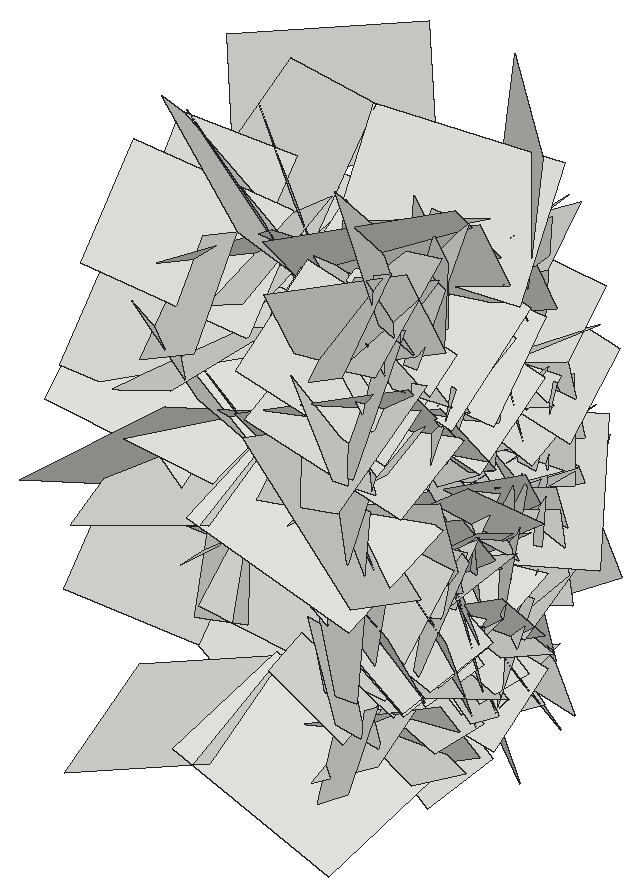
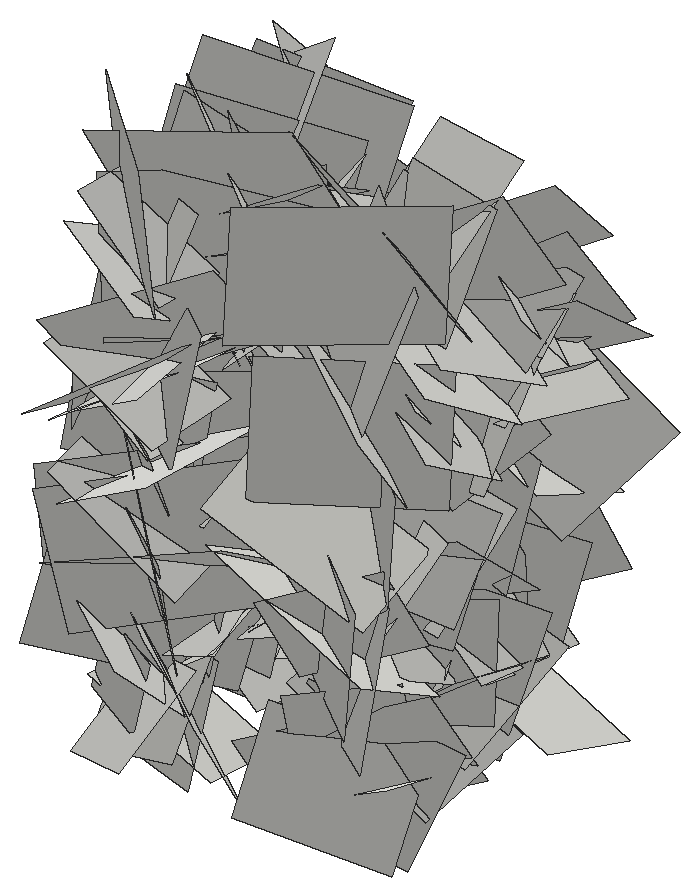
# SketchUp Ruby script. Lengths in inches.
U = 1.inch
M = Sketchup.active_model
def pt(a) = Geom::Point3d.new(a.map { |v| v * U })
def face(e, loops, mat)
  f = e.add_face(loops[0].map { |a| pt(a) })
  loops[1..].each { |l| e.add_face(l.map { |a| pt(a) }).erase! }
  f.material = f.back_material = mat if mat
  f
end
# faces: each face lists its corners as indices into pts; further lists are holes
def faces(e, pts, list, mat = nil) = list.each { |f| face(e, (f[0].is_a?(Array) ? f : [f]).map { |l| l.map { |i| pts[i] } }, mat) }
# xy, xz, yz: faces in a plane at the given z, y or x. An outline is a flat list of corners, or four numbers for a rectangle; further outlines are holes
def ring(l) = l.size == 4 ? [[l[0], l[1]], [l[2], l[1]], [l[2], l[3]], [l[0], l[3]]] : l.each_slice(2).to_a
def flat(e, list, mat, &to3) = list.each { |f| face(e, (f[0].is_a?(Array) ? f : [f]).map { |l| ring(l).map { |u, v| to3.(u, v) } }, mat) }
def xy(e, z, list, mat = nil) = flat(e, list, mat) { |x, y| [x, y, z] }
def xz(e, y, list, mat = nil) = flat(e, list, mat) { |x, z| [x, y, z] }
def yz(e, x, list, mat = nil) = flat(e, list, mat) { |y, z| [x, y, z] }
def lines(e, pts, list) = list.each { |a, b| e.add_line(pt(pts[a]), pt(pts[b])) }
# prism: a flat outline (further loops are holes) pulled along v
def prism(e, loops, v, mat = nil)
  f = face(e, loops, mat); d = Geom::Vector3d.new(v.map { |x| x * U })
  f.pushpull(f.normal.samedirection?(d) ? d.length : -d.length)
end
def box(e, o, s, mat = nil) = prism(e, [[o, [o[0] + s[0], o[1], o[2]], [o[0] + s[0], o[1] + s[1], o[2]], [o[0], o[1] + s[1], o[2]]]], [0, 0, s[2]], mat)
def at(x, y, z, deg = 0) = Geom::Transformation.translation(pt([x, y, z])) * Geom::Transformation.rotation(ORIGIN, Z_AXIS, deg.degrees)
def axes(o, x, y, z) = Geom::Transformation.new([*x, 0, *y, 0, *z, 0, *pt(o).to_a, 1])
def part(name) = M.definitions.add(name)
# library, detail: a bought-in or finely detailed component or shape, given as its bounding box
def library(name, o, s) = part(name).tap { |d| box(d.entities, o, s) }
def detail(e, o, s) = box(e.add_group.entities, o, s)
def put(e, d, t, mat = nil) = e.add_instance(d, t).tap { |i| i.material = mat if mat }
def group(e, t, mat = nil) = e.add_group.tap { |g| g.transformation = t; g.material = mat if mat }.entities
root = M.entities
c1 = part("Component\#6")
p = [[0.01,0,0],[0,3.24,4.54],[4.32,3.24,4.54],[4.33,0,0]]
faces(c1.entities,p,[[0,1,2,3]])
put(root,c1,axes([14.53,167.01,8.33],[0.18631,0.3359,0.73427],[0.04897,0.74605,-0.35235],[0.8545,-0.11599,-0.1399]))
put(root,c1,axes([14.53,166.18,19.56],[-0.12535,0.0531,1.28965],[-0.2192,1.27754,-0.07157],[1.35051,0.21229,0.10808]))
put(root,c1,axes([14.53,168.14,0.12],[-0.06773,-0.63363,0.78179],[0.11595,0.77435,0.63654],[1.06038,-0.12515,-0.01967]))
put(root,c1,axes([14.53,169.19,10.7],[-0.0913,0.46499,-1.24639],[-0.29576,-1.22753,-0.43867],[1.37875,-0.23253,-0.17663]))
put(root,c1,axes([18.5,165.96,10.85],[0.09912,0.20412,-0.70693],[0.02587,-0.71308,-0.20267],[-0.77953,0.00229,-0.09661]))
put(root,c1,axes([18.5,161.25,17.66],[0.25985,0.898,-0.37026],[0.14737,-0.41038,-0.90325],[-1.01902,0.16964,-0.22504]))
put(root,c1,axes([18.5,162.79,15.86],[0.07285,0.46729,0.4905],[-0.02436,0.49435,-0.46773],[-0.71769,0.03066,0.06566]))
put(root,c1,axes([14.53,167.22,15.375],[-0.0235,-0.92066,-0.53568],[-0.01768,-0.53543,0.92093],[1.12894,-0.02755,0.00327]))
put(root,c1,axes([14.53,167.28,17.92],[-0.19972,-0.96368,-0.57877],[0.14667,-0.60226,0.95775],[1.18251,-0.08806,-0.21655]))
put(root,c1,axes([14.53,157.18,19.73],[-0.07599,0.81527,0.8297],[-0.084,0.82592,-0.8184],[1.23014,0.10676,-0.00463]))
put(root,c1,axes([14.53,167.18,1.59],[-0.07507,-1.0991,0.32301],[-0.05871,0.32653,1.09895],[1.2129,-0.05222,0.07319]))
put(root,c1,axes([14.53,168.87,14.79],[0.03205,0.06087,-1.12787],[-0.16204,-1.11767,-0.06442],[1.18627,-0.15431,0.02167]))
put(root,c1,axes([14.53,166.01,11.8],[0.21466,0.53877,-0.68228],[-0.03009,-0.69607,-0.55809],[0.92102,-0.14831,0.14079]))
put(root,c1,axes([14.53,163.57,3.71],[0.11292,-0.2033,0.99476],[-0.09749,0.99417,0.21302],[1.07181,0.11185,-0.08542]))
put(root,c1,axes([14.53,159.91,9.22],[-0.2022,-1.20502,0.50539],[-0.1049,0.52261,1.20871],[1.38114,-0.13672,0.1658]))
put(root,c1,axes([14.53,162.44,14.8125],[-0.22172,-1.13603,-0.19278],[0.19013,-0.22565,1.13507],[1.20652,-0.17321,-0.21429]))
put(root,c1,axes([14.53,160.62,5.12],[0.08568,1.04485,0.18773],[-0.09569,0.19436,-1.04286],[1.1212,-0.06325,-0.10335]))
put(root,c1,axes([18.5,162.91,7.6875],[0.03517,0.6334,0.29771],[0.1292,0.28826,-0.62688],[-0.73053,0.08147,-0.09654]))
put(root,c1,axes([14.53,163.93,5.47],[0.11462,-1.01834,-0.26907],[-0.10191,-0.2789,1.0169],[1.11183,0.07941,0.12095]))
put(root,c1,axes([14.53,156.14,6.5],[0.17845,0.35117,0.84391],[0.01887,0.85668,-0.36003],[0.96872,-0.08137,-0.14844]))
put(root,c1,axes([18.5,170.02,6.34],[0.13634,-0.30577,-0.6303],[0.02329,-0.63876,0.31436],[-0.74222,-0.07621,-0.10592]))
put(root,c1,axes([14.53,160.14,4.78],[0.03826,-0.47304,0.81506],[0.18962,0.80427,0.45886],[0.98077,-0.13704,-0.12051]))
put(root,c1,axes([14.53,166.625,12.7],[0.17127,1.04033,-0.10676],[-0.13463,-0.08771,-1.04688],[1.10034,-0.17266,-0.11147]))
put(root,c1,axes([14.53,168.99,0.33],[0.20008,-0.71049,0.66963],[-0.07161,0.67089,0.73087],[1.03242,0.18422,-0.07908]))
put(root,c1,axes([14.53,164.18,5.53],[0.00871,-1.21515,-0.1589],[-0.11926,-0.15898,1.20995],[1.29354,-0.00648,0.11262]))
put(root,c1,axes([18.5,159.77,13.93],[0.14822,0.47929,0.38572],[-0.01533,0.39801,-0.48932],[-0.65196,0.0996,0.0992]))
put(root,c1,axes([14.53,165.6875,8.33],[0.14254,-0.77018,0.64298],[0.05856,0.65343,0.77114],[1.06187,0.06735,-0.12884]))
put(root,c1,axes([14.53,164.53,2.65],[0.11418,0.95876,0.15487],[0.16789,0.13639,-0.95453],[1.01568,-0.13033,0.14037]))
put(root,c1,axes([14.53,170.79,17.67],[0.07972,-0.69903,-0.88266],[-0.01234,-0.88506,0.69994],[1.19343,0.03754,0.0662]))
put(root,c1,axes([14.53,165.97,13.03],[0.11695,-0.23373,1.15092],[-0.10796,1.14973,0.24325],[1.24018,0.12213,-0.08736]))
put(root,c1,axes([18.5,164.09,3.1],[0.16189,-0.51758,0.36968],[0.06161,0.38995,0.52196],[-0.67139,-0.08902,0.13704]))
put(root,c1,axes([14.53,155.93,16.01],[0.06166,0.77521,1.08886],[-0.24821,1.07895,-0.75564],[1.39492,0.15772,-0.18259]))
put(root,c1,axes([14.53,163.21,2.24],[-0.08398,-0.53221,1.10764],[0.11648,1.10243,0.53756],[1.29738,-0.13342,0.02343]))
put(root,c1,axes([14.53,161.02,12.77],[0.04866,0.36936,-1.04237],[0.12613,-1.03886,-0.36288],[1.16543,0.09701,0.0828]))
put(root,c1,axes([14.53,162.03,18.62],[0.15865,-0.78055,-0.79386],[-0.03617,-0.80384,0.78393],[1.17956,0.08034,0.13081]))
put(root,c1,axes([14.53,161.03,16.77],[-0.02327,0.73455,-0.90907],[0.17416,-0.89826,-0.72978],[1.22657,0.14148,0.08637]))
put(root,c1,axes([14.53,163.86,1.73],[0.03729,0.66749,1.03354],[-0.00972,1.03407,-0.66752],[1.30413,-0.01138,-0.03452]))
put(root,c1,axes([14.53,162.85,15.75],[0.04254,-1.00522,0.67204],[0.02385,0.67292,1.00519],[1.28151,0.02084,-0.04102]))
put(root,c1,axes([14.53,163.36,23.49],[0.04873,0.57368,-1.00395],[0.12423,-1.00188,-0.56714],[1.21936,0.07915,0.09791]))
put(root,c1,axes([14.53,159.69,18.96],[0.02704,0.74145,1.09535],[-0.09362,1.09406,-0.73853],[1.39894,0.05888,-0.07059]))
put(root,c1,axes([14.53,166.4,18.65],[-0.092,-1.19571,-0.63762],[0.0325,-0.6405,1.19693],[1.43603,-0.06211,-0.06794]))
put(root,c1,axes([14.53,155.03,14.95],[-0.10989,1.07322,0.82249],[0.07177,0.82799,-1.07186],[1.43147,0.04087,0.11688]))
put(root,c1,axes([14.53,159.14,18.38],[0.07521,0.79304,-0.86536],[0.12573,-0.86735,-0.78513],[1.23784,0.03991,0.13233]))
put(root,c1,axes([14.53,168.375,23.9],[-0.0952,-0.72561,-1.04974],[0.29336,-1.03837,0.69407],[1.32049,0.17837,-0.22987]))
put(root,c1,axes([14.53,157.93,15.34],[0.27083,1.19165,0.15594],[-0.0802,0.17506,-1.21378],[1.27139,-0.2428,-0.10978]))
put(root,c1,axes([14.53,162.31,11.53],[0.17206,0.75955,-0.87532],[0.12131,-0.89005,-0.75111],[1.22246,-0.01858,0.19774]))
put(root,c1,axes([14.53,165.1,2.71],[-0.06092,-1.21711,0.58199],[0.18306,0.57109,1.21136],[1.41828,-0.12599,-0.13136]))
put(root,c1,axes([14.53,170.58,10.37],[0.24309,-1.14649,0.14454],[0.04952,0.15643,1.16674],[1.2239,0.22139,-0.07591]))
put(root,c1,axes([14.53,161.07,7.88],[0.0926,0.91308,0.78861],[0.24837,0.76278,-0.90913],[1.25453,-0.21841,0.12178]))
put(root,c1,axes([14.53,171.01,11.29],[0.23144,-0.15428,-1.27652],[-0.01824,-1.29503,0.15357],[1.36284,0.00887,0.21884]))
put(root,c1,axes([14.53,167.61,21.95],[0.32344,0.31012,-1.26322],[-0.1451,-1.28265,-0.34796],[1.37111,-0.2089,0.26116]))
put(root,c1,axes([14.53,161.91,24.73],[0.20116,0.87735,-0.9177],[0.06395,-0.93308,-0.87958],[1.34427,-0.0869,0.17917]))
put(root,c1,axes([14.53,161.24,11.55],[0.08722,-1.18104,-0.51149],[0.30261,-0.48302,1.16122],[1.33028,0.18731,-0.23062]))
put(root,c1,axes([14.53,160.65,1.35],[0.1594,-1.22011,-0.46707],[0.28659,-0.43091,1.2127],[1.35486,0.2347,-0.20157]))
put(root,c1,axes([14.53,170.67,8.29],[0.13658,-1.14766,-0.62909],[0.33753,-0.58565,1.13362],[1.34561,0.26339,-0.2205]))
put(root,c1,axes([14.53,161.87,9.58],[0.35888,-0.49511,-1.17449],[0.11741,-1.19919,0.53746],[1.34594,0.23663,0.26628]))
put(root,c1,axes([28.31,161.87,9.58],[-0.35888,-0.49511,-1.17449],[-0.11741,-1.19919,0.53746],[-1.34594,0.23663,0.26628]))
put(root,c1,axes([28.31,170.67,8.29],[-0.13658,-1.14766,-0.62909],[-0.33753,-0.58565,1.13362],[-1.34561,0.26339,-0.2205]))
put(root,c1,axes([28.31,160.65,1.35],[-0.1594,-1.22011,-0.46707],[-0.28659,-0.43091,1.2127],[-1.35486,0.2347,-0.20157]))
put(root,c1,axes([28.31,161.24,11.55],[-0.08722,-1.18104,-0.51149],[-0.30261,-0.48302,1.16122],[-1.33028,0.18731,-0.23062]))
put(root,c1,axes([28.31,161.91,24.73],[-0.20116,0.87735,-0.9177],[-0.06395,-0.93308,-0.87958],[-1.34427,-0.0869,0.17917]))
put(root,c1,axes([28.31,167.61,21.95],[-0.32344,0.31012,-1.26322],[0.1451,-1.28265,-0.34796],[-1.37111,-0.2089,0.26116]))
put(root,c1,axes([28.31,171.01,11.29],[-0.23144,-0.15428,-1.27652],[0.01824,-1.29503,0.15357],[-1.36284,0.00887,0.21884]))
put(root,c1,axes([28.31,161.07,7.88],[-0.0926,0.91308,0.78861],[-0.24837,0.76278,-0.90913],[-1.25453,-0.21841,0.12178]))
put(root,c1,axes([28.31,170.58,10.37],[-0.24309,-1.14649,0.14454],[-0.04952,0.15643,1.16674],[-1.2239,0.22139,-0.07591]))
put(root,c1,axes([28.31,165.1,2.71],[0.06092,-1.21711,0.58199],[-0.18306,0.57109,1.21136],[-1.41828,-0.12599,-0.13136]))
put(root,c1,axes([28.31,162.31,11.53],[-0.17206,0.75955,-0.87532],[-0.12131,-0.89005,-0.75111],[-1.22246,-0.01858,0.19774]))
put(root,c1,axes([28.31,157.93,15.34],[-0.27083,1.19165,0.15594],[0.0802,0.17506,-1.21378],[-1.27139,-0.2428,-0.10978]))
put(root,c1,axes([28.31,168.375,23.9],[0.0952,-0.72561,-1.04974],[-0.29336,-1.03837,0.69407],[-1.32049,0.17837,-0.22987]))
put(root,c1,axes([28.31,159.14,18.38],[-0.07521,0.79304,-0.86536],[-0.12573,-0.86735,-0.78513],[-1.23784,0.03991,0.13233]))
put(root,c1,axes([28.31,155.03,14.95],[0.10989,1.07322,0.82249],[-0.07177,0.82799,-1.07186],[-1.43147,0.04087,0.11688]))
put(root,c1,axes([28.31,166.4,18.65],[0.092,-1.19571,-0.63762],[-0.0325,-0.6405,1.19693],[-1.43603,-0.06211,-0.06794]))
put(root,c1,axes([28.31,159.69,18.96],[-0.02704,0.74145,1.09535],[0.09362,1.09406,-0.73853],[-1.39894,0.05888,-0.07059]))
put(root,c1,axes([28.31,163.36,23.49],[-0.04873,0.57368,-1.00395],[-0.12423,-1.00188,-0.56714],[-1.21936,0.07915,0.09791]))
put(root,c1,axes([28.31,162.85,15.75],[-0.04254,-1.00522,0.67204],[-0.02385,0.67292,1.00519],[-1.28151,0.02084,-0.04102]))
put(root,c1,axes([28.31,163.86,1.73],[-0.03729,0.66749,1.03354],[0.00972,1.03407,-0.66752],[-1.30413,-0.01138,-0.03452]))
put(root,c1,axes([28.31,161.03,16.77],[0.02327,0.73455,-0.90907],[-0.17416,-0.89826,-0.72978],[-1.22657,0.14148,0.08637]))
put(root,c1,axes([28.31,162.03,18.62],[-0.15865,-0.78055,-0.79386],[0.03617,-0.80384,0.78393],[-1.17956,0.08034,0.13081]))
put(root,c1,axes([28.31,161.02,12.77],[-0.04866,0.36936,-1.04237],[-0.12613,-1.03886,-0.36288],[-1.16543,0.09701,0.0828]))
put(root,c1,axes([28.31,163.21,2.24],[0.08398,-0.53221,1.10764],[-0.11648,1.10243,0.53756],[-1.29738,-0.13342,0.02343]))
put(root,c1,axes([28.31,155.93,16.01],[-0.06166,0.77521,1.08886],[0.24821,1.07895,-0.75564],[-1.39492,0.15772,-0.18259]))
put(root,c1,axes([24.34,164.09,3.1],[-0.16189,-0.51758,0.36968],[-0.06161,0.38995,0.52196],[0.67139,-0.08902,0.13704]))
put(root,c1,axes([28.31,165.97,13.03],[-0.11695,-0.23373,1.15092],[0.10796,1.14973,0.24325],[-1.24018,0.12213,-0.08736]))
put(root,c1,axes([28.31,170.79,17.67],[-0.07972,-0.69903,-0.88266],[0.01234,-0.88506,0.69994],[-1.19343,0.03754,0.0662]))
put(root,c1,axes([24.34,155.94,6.59],[-0.14653,0.65267,0.04592],[-0.0729,0.03218,-0.6644],[0.6897,0.14207,-0.06047]))
put(root,c1,axes([28.31,164.53,2.65],[-0.11418,0.95876,0.15487],[-0.16789,0.13639,-0.95453],[-1.01568,-0.13033,0.14037]))
put(root,c1,axes([28.31,165.6875,8.33],[-0.14254,-0.77018,0.64298],[-0.05856,0.65343,0.77114],[-1.06187,0.06735,-0.12884]))
put(root,c1,axes([24.34,159.77,13.93],[-0.14822,0.47929,0.38572],[0.01533,0.39801,-0.48932],[0.65196,0.0996,0.0992]))
put(root,c1,axes([28.31,164.18,5.53],[-0.00871,-1.21515,-0.1589],[0.11926,-0.15898,1.20995],[-1.29354,-0.00648,0.11262]))
put(root,c1,axes([28.31,168.99,0.33],[-0.20008,-0.71049,0.66963],[0.07161,0.67089,0.73087],[-1.03242,0.18422,-0.07908]))
put(root,c1,axes([28.31,166.625,12.7],[-0.17127,1.04033,-0.10676],[0.13463,-0.08771,-1.04688],[-1.10034,-0.17266,-0.11147]))
put(root,c1,axes([28.31,160.14,4.78],[-0.03826,-0.47304,0.81506],[-0.18962,0.80427,0.45886],[-0.98077,-0.13704,-0.12051]))
put(root,c1,axes([24.34,170.02,6.34],[-0.13634,-0.30577,-0.6303],[-0.02329,-0.63876,0.31436],[0.74222,-0.07621,-0.10592]))
put(root,c1,axes([28.31,156.14,6.5],[-0.17845,0.35117,0.84391],[-0.01887,0.85668,-0.36003],[-0.96872,-0.08137,-0.14844]))
put(root,c1,axes([28.31,163.93,5.47],[-0.11462,-1.01834,-0.26907],[0.10191,-0.2789,1.0169],[-1.11183,0.07941,0.12095]))
put(root,c1,axes([24.34,162.91,7.6875],[-0.03517,0.6334,0.29771],[-0.1292,0.28826,-0.62688],[0.73053,0.08147,-0.09654]))
put(root,c1,axes([28.31,160.62,5.12],[-0.08568,1.04485,0.18773],[0.09569,0.19436,-1.04286],[-1.1212,-0.06325,-0.10335]))
put(root,c1,axes([28.31,162.44,14.8125],[0.22172,-1.13603,-0.19278],[-0.19013,-0.22565,1.13507],[-1.20652,-0.17321,-0.21429]))
put(root,c1,axes([28.31,159.91,9.22],[0.2022,-1.20502,0.50539],[0.1049,0.52261,1.20871],[-1.38114,-0.13672,0.1658]))
put(root,c1,axes([28.31,163.57,3.71],[-0.11292,-0.2033,0.99476],[0.09749,0.99417,0.21302],[-1.07181,0.11185,-0.08542]))
put(root,c1,axes([28.31,166.01,11.8],[-0.21466,0.53877,-0.68228],[0.03009,-0.69607,-0.55809],[-0.92102,-0.14831,0.14079]))
put(root,c1,axes([28.31,168.87,14.79],[-0.03205,0.06087,-1.12787],[0.16204,-1.11767,-0.06442],[-1.18627,-0.15431,0.02167]))
put(root,c1,axes([28.31,167.18,1.59],[0.07507,-1.0991,0.32301],[0.05871,0.32653,1.09895],[-1.2129,-0.05222,0.07319]))
put(root,c1,axes([28.31,157.18,19.73],[0.07599,0.81527,0.8297],[0.084,0.82592,-0.8184],[-1.23014,0.10676,-0.00463]))
put(root,c1,axes([28.31,167.28,17.92],[0.19972,-0.96368,-0.57877],[-0.14667,-0.60226,0.95775],[-1.18251,-0.08806,-0.21655]))
put(root,c1,axes([28.31,167.22,15.375],[0.0235,-0.92066,-0.53568],[0.01768,-0.53543,0.92093],[-1.12894,-0.02755,0.00327]))
put(root,c1,axes([24.34,162.79,15.86],[-0.07285,0.46729,0.4905],[0.02436,0.49435,-0.46773],[0.71769,0.03066,0.06566]))
put(root,c1,axes([24.34,161.25,17.66],[-0.25985,0.898,-0.37026],[-0.14737,-0.41038,-0.90325],[1.01902,0.16964,-0.22504]))
put(root,c1,axes([24.34,165.96,10.85],[-0.09912,0.20412,-0.70693],[-0.02587,-0.71308,-0.20267],[0.77953,0.00229,-0.09661]))
put(root,c1,axes([28.31,169.19,10.7],[0.0913,0.46499,-1.24639],[0.29576,-1.22753,-0.43867],[-1.37875,-0.23253,-0.17663]))
put(root,c1,axes([28.31,168.14,0.12],[0.06773,-0.63363,0.78179],[-0.11595,0.77435,0.63654],[-1.06038,-0.12515,-0.01967]))
put(root,c1,axes([28.31,166.18,19.56],[0.12535,0.0531,1.28965],[0.2192,1.27754,-0.07157],[-1.35051,0.21229,0.10808]))
put(root,c1,axes([28.31,167.01,8.33],[-0.18631,0.3359,0.73427],[-0.04897,0.74605,-0.35235],[-0.8545,-0.11599,-0.1399]))
put(root,c1,axes([24.34,159.82,10.86],[-0.164,0.05549,-0.7166],[0.119,-0.72215,-0.08015],[0.75252,0.12629,-0.14349]))
put(root,c1,axes([28.31,164.72,6.23],[0.02586,0.29335,1.1723],[0.23754,1.1511,-0.29271],[-1.25874,0.22326,-0.03115]))
put(root,c1,axes([24.34,164.71,11.17],[-0.09162,-0.23701,0.75882],[-0.09076,0.76162,0.22813],[0.83777,0.05659,0.1077]))
put(root,c1,axes([24.34,167.39,12.19],[-0.06725,0.11282,-0.6237],[0.12717,-0.61335,-0.12315],[0.65971,0.12973,-0.03984]))
put(root,c1,axes([24.34,158.25,7.85],[0.01053,0.60228,-0.51533],[-0.19634,-0.49934,-0.58716],[0.81696,-0.12777,-0.13447]))
put(root,c1,axes([28.31,165.51,17.74],[-0.00528,-0.97827,-0.44464],[0.11526,-0.44282,0.97306],[-1.13321,-0.04048,0.10104]))
put(root,c1,axes([28.31,165.75,-1.09],[0.03685,-0.4153,0.96157],[0.02645,0.96216,0.41465],[-1.10996,0.00914,0.04181]))
put(root,c1,axes([28.31,167.74,3.51],[0.11337,-0.86322,0.3774],[-0.28126,0.33685,0.84566],[-0.95821,-0.201,-0.20357]))
put(root,c1,axes([28.31,161.03,4.22],[-0.00206,0.54706,-0.73945],[-0.10036,-0.73565,-0.544],[-0.96983,0.07497,0.05787]))
put(root,c1,axes([28.31,158.84,13.7],[-0.15038,-0.75335,0.50607],[0.08727,0.49942,0.76653],[-0.95804,0.16374,-0.00961]))
put(root,c1,axes([28.31,166.72,20.27],[-0.14718,0.45385,-0.66356],[-0.05291,-0.67695,-0.45256],[-0.85051,-0.03642,0.14299]))
put(root,c1,axes([24.34,158.82,19.64],[0.09205,0.73549,-0.019],[-0.17536,0.00088,-0.72213],[0.75991,-0.08889,-0.16434]))
put(root,c1,axes([28.31,169.09,13.37],[-0.12805,-0.81492,0.2825],[0.01832,0.28292,0.8235],[-0.91406,0.11983,-0.02307]))
put(root,c1,axes([24.34,159.61,12.59],[0.0897,0.16152,-0.57424],[0.01993,-0.58042,-0.16049],[0.632,-0.00462,0.08656]))
put(root,c1,axes([24.34,160.65,18.69],[0.1336,-0.1743,0.59472],[-0.06624,0.60023,0.18916],[0.65357,0.09646,-0.1024]))
put(root,c1,axes([24.34,160.54,14.42],[-0.065,-0.29459,-0.75204],[-0.0763,-0.74921,0.29935],[0.85274,-0.0895,-0.03054]))
put(root,c1,axes([24.34,161.26,10.83],[-0.08958,0.45503,-0.59155],[0.06652,-0.58889,-0.46195],[0.78829,0.10141,-0.02824]))
put(root,c1,axes([28.31,170.16,13.55],[0.14984,-1.04824,-0.22204],[-0.00627,-0.22472,1.05715],[-1.13577,-0.13705,-0.03513]))
put(root,c1,axes([24.34,160.97,6.7],[0.04912,0.73058,0.10133],[-0.09877,0.10652,-0.72536],[0.77557,-0.03271,-0.0988]))
put(root,c1,axes([28.31,163.26,10.51],[-0.09772,0.8385,-0.3881],[0.10419,-0.37892,-0.842],[-0.97385,-0.12468,-0.05114]))
put(root,c1,axes([24.34,159.79,25.07],[-0.1328,0.69586,-0.68383],[-0.18687,-0.69425,-0.67416],[1.01714,-0.03669,-0.21313]))
put(root,c1,axes([28.31,167.39,3.05],[0.22625,-1.02118,-0.283],[-0.12014,-0.30902,1.02962],[-1.11681,-0.17363,-0.16809]))
put(root,c1,axes([24.34,159.32,12.84],[0.06752,-0.16321,-0.59207],[0.0871,-0.58763,0.17083],[0.64514,0.09641,0.0389]))
put(root,c1,axes([24.34,169.73,5.36],[0.07377,0.11031,-0.61615],[0.06228,-0.61836,-0.10407],[0.66058,0.04598,0.07863]))
put(root,c1,axes([28.31,166.22,16.78],[0.0558,0.90138,-0.08554],[-0.09664,-0.07998,-0.89882],[-0.95488,0.06076,0.08597]))
put(root,c1,axes([24.34,166.8,6.58],[-0.19077,-0.84984,-0.315],[0.00737,-0.32244,0.86593],[0.9607,-0.16629,-0.0692]))
put(root,c1,axes([28.31,159.03,23.29],[0.13252,0.38295,-0.87838],[-0.10893,-0.87536,-0.39626],[-1.00987,0.14467,-0.07253]))
put(root,c1,axes([24.34,160.57,3.12],[0.03509,0.82869,0.13415],[-0.15764,0.13792,-0.81528],[0.87577,-0.00838,-0.15213]))
put(root,c1,axes([24.34,164.04,15.7],[0.03624,-0.6234,-0.24842],[0.08,-0.24359,0.62167],[0.70683,0.05954,-0.05762]))
put(root,c1,axes([28.31,170.98,12.21],[0.31631,-0.51758,-1.19288],[0.16648,-1.20059,0.56021],[-1.36826,-0.26573,-0.20761]))
put(root,c1,axes([24.34,169.83,13.22],[0.13817,-0.64015,-0.16037],[-0.03989,-0.17041,0.64965],[0.69839,0.11692,0.06883]))
put(root,c1,axes([24.34,161.46,7.67],[0.11157,-0.00104,0.59962],[0.09459,0.60203,-0.01462],[0.62852,-0.09042,-0.10424]))
put(root,c1,axes([28.31,168.08,9.41],[0.11593,0.02752,-0.90523],[-0.14705,-0.90054,-0.04413],[-0.94866,0.14295,-0.10378]))
put(root,c1,axes([24.34,169.26,18.83],[0.02849,-0.83115,-0.05333],[-0.13283,-0.05679,0.82186],[0.87278,0.01849,0.12683]))
put(root,c1,axes([24.34,165.55,15.88],[-0.02597,-0.35934,-0.67832],[0.02345,-0.67872,0.35875],[0.81334,0.00809,-0.032]))
put(root,c1,axes([24.34,167.12,21.5],[0.0656,0.35319,-0.61189],[0.00255,-0.61434,-0.35436],[0.7489,-0.02885,0.0548]))
put(root,c1,axes([28.31,164.04,2.37],[0.08884,-0.86849,0.07962],[-0.14736,0.06566,0.86256],[-0.91264,-0.09515,-0.13152]))
put(root,c1,axes([28.31,162.54,0.74],[0.05881,-0.79857,0.25436],[-0.14334,0.24305,0.79255],[-0.87675,-0.0933,-0.11251]))
put(root,c1,axes([28.31,157.37,3.29],[-0.12325,0.67494,0.21472],[-0.06797,0.20667,-0.68436],[-0.74769,-0.13004,0.02682]))
put(root,c1,axes([28.31,166.02,4.84],[0.16866,0.71959,0.68076],[-0.0323,0.69272,-0.72511],[-1.04952,0.09433,0.13172]))
put(root,c1,axes([24.34,162.4,12.14],[0.15913,-0.1111,0.71617],[-0.10617,0.72117,0.13287],[0.76084,0.12387,-0.13124]))
put(root,c1,axes([24.34,165.06,16.01],[-0.24936,0.99659,0.4051],[-0.07669,0.39908,-1.02378],[1.13774,0.24532,0.01978]))
put(root,c1,axes([24.34,164.7,6.68],[-0.19863,-0.78204,0.62344],[-0.03401,0.63866,0.7915],[1.0596,-0.1261,0.14227]))
put(root,c1,axes([28.31,166.67,11.65],[-0.03639,0.32382,0.70516],[-0.0632,0.70266,-0.32558],[-0.82009,-0.06852,-0.0062]))
put(root,c1,axes([28.31,166.25,3.34],[-0.10377,-0.78092,-0.09398],[0.04515,-0.09983,0.78516],[-0.83253,0.09192,0.05429]))
put(root,c1,axes([28.31,167.84,10.46],[0.01526,0.23241,-0.73689],[-0.14958,-0.72384,-0.23105],[-0.80526,0.13886,0.02896]))
put(root,c1,axes([28.31,164.66,7.18],[0.03191,0.54978,-0.59147],[-0.106,-0.58478,-0.54866],[-0.84939,0.09364,0.04625]))
put(root,c1,axes([28.31,155.24,20.59],[-0.01301,0.69003,0.71111],[0.211,0.69839,-0.67424],[-1.02891,0.13449,-0.14726]))
put(root,c1,axes([28.31,167.39,19.82],[-0.12929,0.6108,0.35138],[-0.02449,0.35295,-0.62154],[-0.74654,-0.11736,-0.04046]))
put(root,c1,axes([24.34,165.07,9.38],[0.13081,0.27606,-0.70722],[-0.08788,-0.70731,-0.29057],[0.79993,-0.12284,0.08373]))
put(root,c1,axes([28.31,159.79,6],[0.13547,0.51146,0.93772],[0.15367,0.92736,-0.52557],[-1.12174,0.18881,0.04125]))
put(root,c1,axes([28.31,159.9,13.67],[0.02397,0.44215,0.82689],[0.11898,0.8199,-0.44149],[-0.98679,0.1096,-0.03314]))
put(root,c1,axes([24.34,164.44,22.83],[-0.02931,-0.02413,-0.88007],[-0.04764,-0.87932,0.02552],[0.93201,-0.0457,-0.02637]))
put(root,c1,axes([28.31,168.54,15.47],[0.051,0.16682,-0.79913],[-0.09039,-0.79511,-0.17112],[-0.86061,0.0934,-0.02938]))
put(root,c1,axes([28.31,155.625,2.89],[-0.13104,0.56412,0.5606],[0.11872,0.57403,-0.55293],[-0.83462,-0.00692,-0.16667]))
